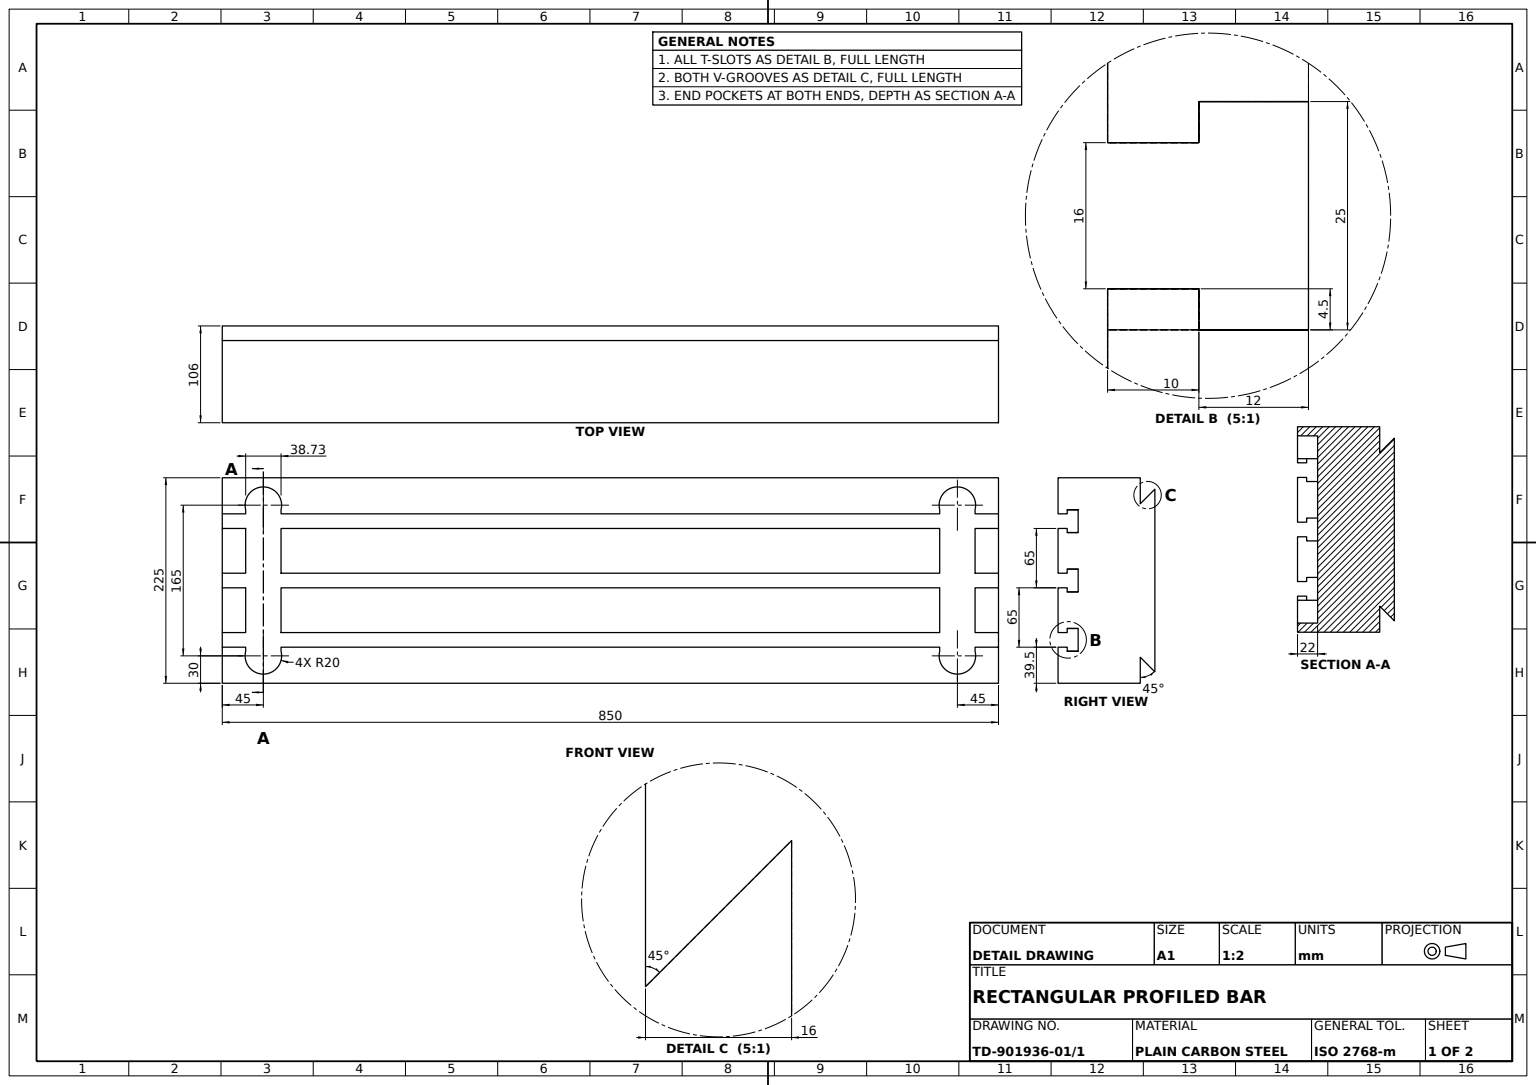
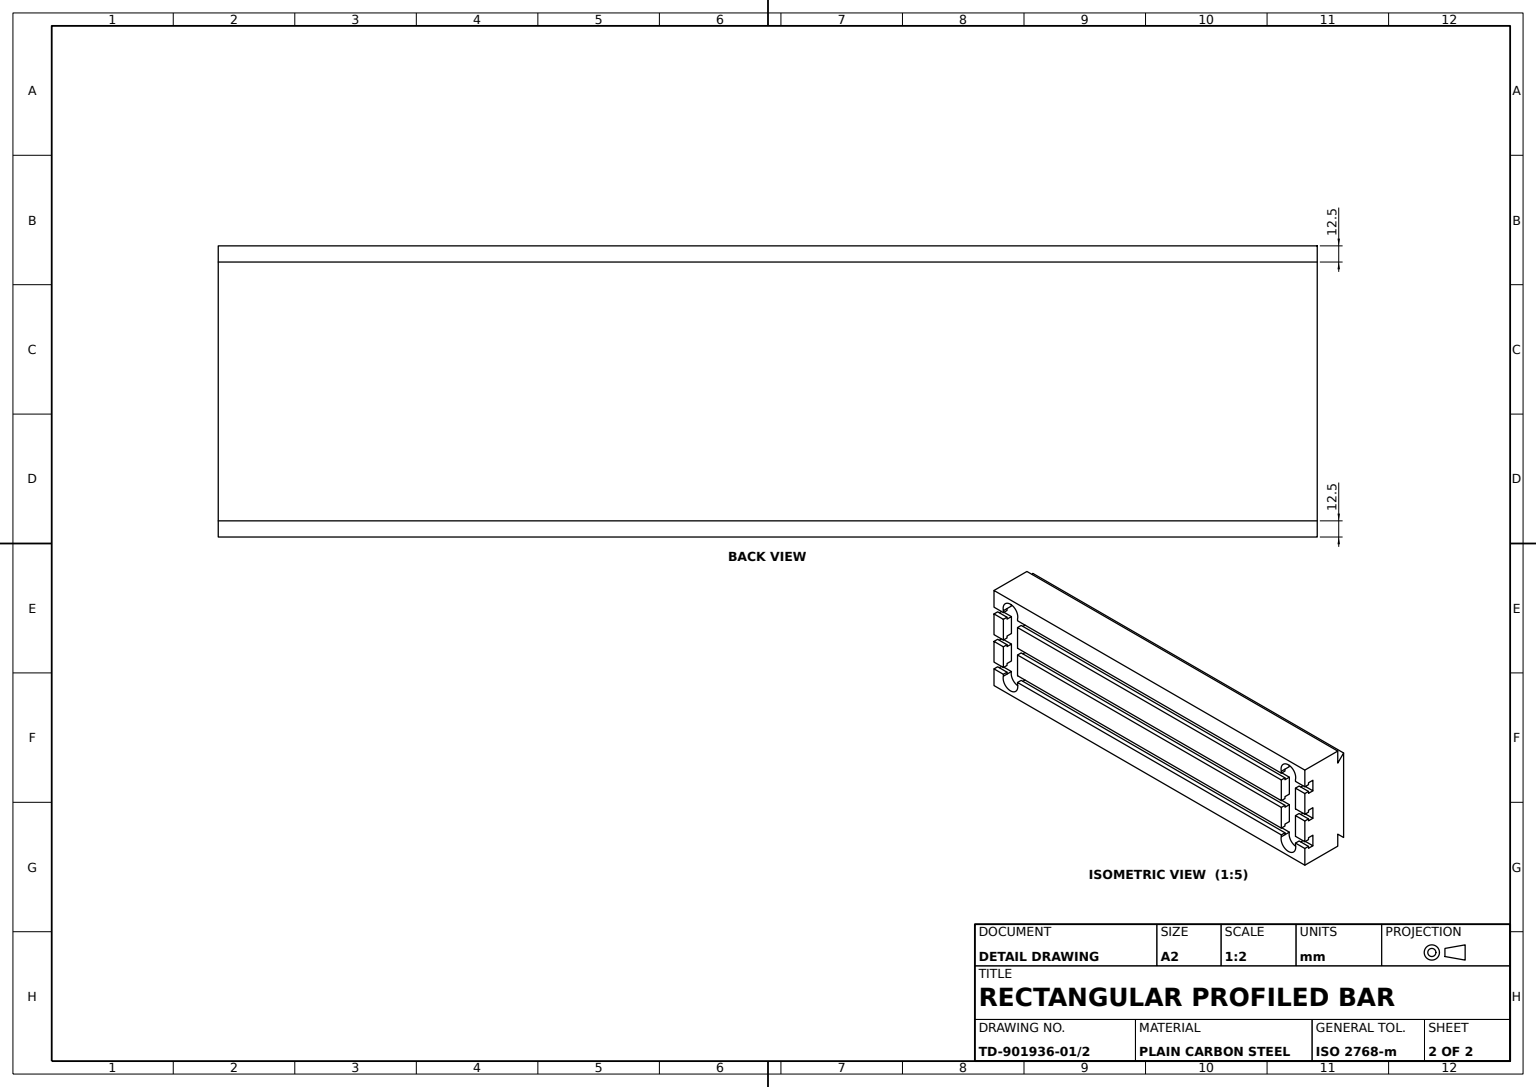
solid
v1 (-400,82.5,106)
v2 (-399.363172,77.493249,106)
e1 v1 v2 CIRCLE(AX(P(-380,82.5,106),D(0,0,1),D(1,0,0)),20)
v3 (-399.363172,77.493249,96)
e2 v3 v2 LINE
v4 (-399.364917,77.5,96)
e3 v4 v3 CIRCLE(AX(P(-380,82.5,96),D(0,0,1),D(1,0,0)),20)
v5 (-399.364917,77.5,84)
e4 v5 v4 LINE
v6 (-400,82.5,84)
e5 v6 v5 CIRCLE(AX(P(-380,82.5,84),D(0,0,1),D(-1,0,0)),20)
e6 v6 v1 LINE
face CYL(AX(P(-380,82.5,-124.865986),D(0,0,1),D(1,0,0)),20) rev [e1 -e2 -e3 -e4 -e5 e6]
v7 (360.635083,-77.5,96)
v8 (360.635083,-77.5,84)
e7 v7 v8 LINE
v9 (-360.635083,-77.5,84)
e8 v9 v8 LINE
v10 (-360.635083,-77.5,96)
e9 v9 v10 LINE
e10 v10 v7 LINE
face PLANE(AX(P(-425,-77.5,96),D(0,-1,0),D(0,0,-1))) rev [e7 -e8 e9 e10]
v11 (-400,-82.5,106)
v12 (-360,-82.5,106)
e11 v11 v12 CIRCLE(AX(P(-380,-82.5,106),D(0,0,1),D(1,0,0)),20)
v13 (-399.363172,-77.493249,106)
e12 v13 v11 CIRCLE(AX(P(-380,-82.5,106),D(0,0,1),D(1,0,0)),20)
v14 (-399.363172,-73,106)
e13 v14 v13 LINE
v15 (-425,-73,106)
e14 v15 v14 LINE
v16 (-425,-112.5,106)
e15 v15 v16 LINE
v17 (425,-112.5,106)
e16 v16 v17 LINE
v18 (425,-73,106)
e17 v17 v18 LINE
v19 (399.363172,-73,106)
e18 v19 v18 LINE
v20 (399.363172,-77.493249,106)
e19 v20 v19 LINE
v21 (400,-82.5,106)
e20 v21 v20 CIRCLE(AX(P(380,-82.5,106),D(0,0,1),D(-1,0,0)),20)
v22 (360,-82.5,106)
e21 v22 v21 CIRCLE(AX(P(380,-82.5,106),D(0,0,1),D(-1,0,0)),20)
v23 (360.636828,-77.493249,106)
e22 v23 v22 CIRCLE(AX(P(380,-82.5,106),D(0,0,1),D(-1,0,0)),20)
v24 (360.636828,-73,106)
e23 v24 v23 LINE
v25 (-360.636828,-73,106)
e24 v25 v24 LINE
v26 (-360.636828,-77.493249,106)
e25 v26 v25 LINE
e26 v12 v26 CIRCLE(AX(P(-380,-82.5,106),D(0,0,1),D(1,0,0)),20)
face PLANE(AX(P(0,0,106),D(0,0,1),D(1,0,0))) [-e11 -e12 -e13 -e14 e15 e16 e17 -e18 -e19 -e20 -e21 -e22 -e23 -e24 -e25 -e26]
v27 (-425,-8,106)
v28 (-425,-57,106)
e27 v27 v28 LINE
v29 (-425,-8,96)
e28 v27 v29 LINE
v30 (-425,-12.5,96)
e29 v29 v30 LINE
v31 (-425,-12.5,84)
e30 v30 v31 LINE
v32 (-425,12.5,84)
e31 v31 v32 LINE
v33 (-425,12.5,96)
e32 v32 v33 LINE
v34 (-425,8,96)
e33 v33 v34 LINE
v35 (-425,8,106)
e34 v34 v35 LINE
v36 (-425,57,106)
e35 v36 v35 LINE
v37 (-425,57,96)
e36 v36 v37 LINE
v38 (-425,52.5,96)
e37 v37 v38 LINE
v39 (-425,52.5,84)
e38 v38 v39 LINE
v40 (-425,77.5,84)
e39 v39 v40 LINE
v41 (-425,77.5,96)
e40 v40 v41 LINE
v42 (-425,73,96)
e41 v41 v42 LINE
v43 (-425,73,106)
e42 v42 v43 LINE
v44 (-425,112.5,106)
e43 v44 v43 LINE
v45 (-425,112.5,16)
e44 v44 v45 LINE
v46 (-425,84,16)
e45 v45 v46 LINE
v47 (-425,100,0)
e46 v46 v47 LINE
v48 (-425,-100,0)
e47 v47 v48 LINE
v49 (-425,-84,16)
e48 v48 v49 LINE
v50 (-425,-112.5,16)
e49 v49 v50 LINE
e50 v16 v50 LINE
v51 (-425,-73,96)
e51 v15 v51 LINE
v52 (-425,-77.5,96)
e52 v51 v52 LINE
v53 (-425,-77.5,84)
e53 v52 v53 LINE
v54 (-425,-52.5,84)
e54 v53 v54 LINE
v55 (-425,-52.5,96)
e55 v54 v55 LINE
v56 (-425,-57,96)
e56 v55 v56 LINE
e57 v56 v28 LINE
face PLANE(AX(P(-425,-112.5,106),D(1,0,0),D(0,0,-1))) rev [-e27 e28 e29 e30 e31 e32 e33 e34 -e35 e36 e37 e38 e39 e40 e41 e42 -e43 e44 e45 e46 e47 e48 e49 -e50 -e15 e51 e52 e53 e54 e55 e56 e57]
v57 (399.363172,-12.5,96)
v58 (399.363172,-8,96)
e58 v57 v58 LINE
v59 (425,-8,96)
e59 v58 v59 LINE
v60 (425,-12.5,96)
e60 v59 v60 LINE
e61 v57 v60 LINE
face PLANE(AX(P(-425,-8,96),D(0,0,1),D(1,0,0))) rev [e58 e59 e60 -e61]
v61 (425,-84,16)
e62 v49 v61 LINE
v62 (425,-112.5,16)
e63 v61 v62 LINE
e64 v50 v62 LINE
face PLANE(AX(P(-425,-84,16),D(0,0,1),D(0,-1,0))) rev [-e49 e62 e63 -e64]
v63 (-360,-82.5,84)
e65 v63 v12 LINE
v64 (-400,-82.5,84)
e66 v64 v63 CIRCLE(AX(P(-380,-82.5,84),D(0,0,1),D(-1,0,0)),20)
e67 v64 v11 LINE
face CYL(AX(P(-380,-82.5,-124.865986),D(0,0,1),D(1,0,0)),20) rev [e11 -e65 -e66 e67]
v65 (-399.364917,-77.5,96)
e68 v52 v65 LINE
v66 (-399.364917,-77.5,84)
e69 v65 v66 LINE
e70 v53 v66 LINE
face PLANE(AX(P(-425,-77.5,96),D(0,-1,0),D(0,0,-1))) rev [e68 e69 -e70 -e53]
e71 v17 v62 LINE
face PLANE(AX(P(425,-112.5,106),D(0,1,0),D(-1,0,0))) rev [e50 e64 -e71 -e16]
v67 (-399.363172,73,96)
e72 v3 v67 LINE
v68 (-399.363172,73,106)
e73 v2 v68 LINE
e74 v67 v68 LINE
face PLANE(AX(P(-399.363172,-77.493249,-124.865986),D(-1,0,0),D(0,0,1))) rev [-e72 e2 e73 -e74]
v69 (399.363172,73,96)
v70 (399.363172,77.493249,96)
e75 v69 v70 LINE
v71 (399.364917,77.5,96)
e76 v70 v71 CIRCLE(AX(P(380,82.5,96),D(0,0,1),D(1,0,0)),20)
v72 (425,77.5,96)
e77 v71 v72 LINE
v73 (425,73,96)
e78 v72 v73 LINE
e79 v69 v73 LINE
face PLANE(AX(P(-425,73,96),D(0,0,1),D(1,0,0))) rev [e75 e76 e77 e78 -e79]
v74 (399.363172,57,96)
v75 (425,57,96)
e80 v74 v75 LINE
v76 (399.363172,57,106)
e81 v74 v76 LINE
v77 (425,57,106)
e82 v76 v77 LINE
e83 v77 v75 LINE
face PLANE(AX(P(-425,57,106),D(0,-1,0),D(0,0,-1))) rev [-e80 e81 e82 e83]
v78 (360.636828,57,106)
v79 (360.636828,8,106)
e84 v78 v79 LINE
v80 (360.636828,8,96)
e85 v80 v79 LINE
v81 (360.636828,12.5,96)
e86 v81 v80 LINE
v82 (360.636828,12.5,84)
e87 v82 v81 LINE
v83 (360.636828,52.5,84)
e88 v83 v82 LINE
v84 (360.636828,52.5,96)
e89 v84 v83 LINE
v85 (360.636828,57,96)
e90 v85 v84 LINE
e91 v78 v85 LINE
face PLANE(AX(P(360.636828,-77.493249,-124.865986),D(-1,0,0),D(0,0,1))) rev [e84 -e85 -e86 -e87 -e88 -e89 -e90 -e91]
v86 (360.636828,-77.493249,96)
e92 v86 v23 LINE
v87 (360.636828,-73,96)
e93 v87 v86 LINE
e94 v24 v87 LINE
face PLANE(AX(P(360.636828,-77.493249,-124.865986),D(-1,0,0),D(0,0,1))) rev [e23 -e92 -e93 -e94]
v88 (399.363172,-52.5,84)
v89 (425,-52.5,84)
e95 v88 v89 LINE
v90 (425,-52.5,96)
e96 v89 v90 LINE
v91 (399.363172,-52.5,96)
e97 v91 v90 LINE
e98 v91 v88 LINE
face PLANE(AX(P(-425,-52.5,96),D(0,1,0),D(0,0,1))) rev [e95 e96 -e97 e98]
v92 (-399.363172,8,96)
e99 v34 v92 LINE
v93 (-399.363172,8,106)
e100 v92 v93 LINE
e101 v35 v93 LINE
face PLANE(AX(P(-425,8,106),D(0,1,0),D(0,0,1))) rev [e99 e100 -e101 -e34]
v94 (425,12.5,96)
v95 (425,8,96)
e102 v94 v95 LINE
v96 (399.363172,8,96)
e103 v96 v95 LINE
v97 (399.363172,12.5,96)
e104 v96 v97 LINE
e105 v97 v94 LINE
face PLANE(AX(P(-425,8,96),D(0,0,1),D(1,0,0))) rev [e102 -e103 e104 e105]
v98 (425,112.5,16)
v99 (425,84,16)
e106 v98 v99 LINE
e107 v46 v99 LINE
e108 v45 v98 LINE
face PLANE(AX(P(-425,84,16),D(0,0,1),D(0,-1,0))) rev [e106 -e107 -e45 e108]
v100 (425,52.5,96)
e109 v75 v100 LINE
v101 (399.363172,52.5,96)
e110 v101 v100 LINE
e111 v101 v74 LINE
face PLANE(AX(P(-425,57,96),D(0,0,1),D(1,0,0))) rev [e109 -e110 e111 e80]
v102 (360.636828,-8,96)
v103 (360.636828,-12.5,96)
e112 v102 v103 LINE
v104 (-360.636828,-12.5,96)
e113 v104 v103 LINE
v105 (-360.636828,-8,96)
e114 v104 v105 LINE
e115 v105 v102 LINE
face PLANE(AX(P(-425,-8,96),D(0,0,1),D(1,0,0))) rev [e112 -e113 e114 e115]
v106 (-399.363172,-77.493249,96)
e116 v106 v13 LINE
e117 v66 v64 CIRCLE(AX(P(-380,-82.5,84),D(0,0,1),D(-1,0,0)),20)
e118 v106 v65 CIRCLE(AX(P(-380,-82.5,96),D(0,0,1),D(1,0,0)),20)
face CYL(AX(P(-380,-82.5,-124.865986),D(0,0,1),D(1,0,0)),20) rev [e116 e12 -e67 -e117 -e69 -e118]
v107 (400,82.5,84)
v108 (400,82.5,106)
e119 v107 v108 LINE
v109 (360,82.5,106)
e120 v108 v109 CIRCLE(AX(P(380,82.5,106),D(0,0,1),D(-1,0,0)),20)
v110 (360,82.5,84)
e121 v110 v109 LINE
e122 v107 v110 CIRCLE(AX(P(380,82.5,84),D(0,0,1),D(-1,0,0)),20)
face CYL(AX(P(380,82.5,-124.865986),D(0,0,1),D(1,0,0)),20) rev [e119 e120 -e121 -e122]
v111 (425,100,0)
e123 v99 v111 LINE
e124 v47 v111 LINE
face PLANE(AX(P(-425,100,0),D(0,-0.707106781,-0.707106781),D(0,0.707106781,-0.707106781))) rev [-e46 e107 e123 -e124]
v112 (-399.363172,57,106)
e125 v112 v93 LINE
e126 v36 v112 LINE
face PLANE(AX(P(0,0,106),D(0,0,1),D(1,0,0))) [e101 -e125 -e126 e35]
v113 (-399.363172,-8,96)
e127 v29 v113 LINE
v114 (-399.363172,-12.5,96)
e128 v113 v114 LINE
e129 v30 v114 LINE
face PLANE(AX(P(-425,-8,96),D(0,0,1),D(1,0,0))) rev [e127 e128 -e129 -e29]
v115 (-360.636828,57,106)
e130 v115 v78 LINE
v116 (-360.636828,8,106)
e131 v116 v115 LINE
e132 v116 v79 LINE
face PLANE(AX(P(0,0,106),D(0,0,1),D(1,0,0))) [-e130 -e131 e132 -e84]
v117 (360,-82.5,84)
e133 v117 v22 LINE
e134 v8 v117 CIRCLE(AX(P(380,-82.5,84),D(0,0,1),D(-1,0,0)),20)
e135 v86 v7 CIRCLE(AX(P(380,-82.5,96),D(0,0,1),D(1,0,0)),20)
face CYL(AX(P(380,-82.5,-124.865986),D(0,0,1),D(1,0,0)),20) rev [e22 -e133 -e134 -e7 -e135 e92]
v118 (-360.636828,-12.5,84)
v119 (360.636828,-12.5,84)
e136 v118 v119 LINE
e137 v118 v104 LINE
e138 v103 v119 LINE
face PLANE(AX(P(-425,-12.5,96),D(0,-1,0),D(0,0,-1))) rev [-e136 e137 e113 e138]
v120 (-360.636828,8,96)
e139 v120 v80 LINE
v121 (-360.636828,12.5,96)
e140 v120 v121 LINE
e141 v121 v81 LINE
face PLANE(AX(P(-425,8,96),D(0,0,1),D(1,0,0))) rev [e86 -e139 e140 e141]
v122 (425,-100,0)
e142 v122 v61 LINE
e143 v48 v122 LINE
face PLANE(AX(P(-425,-100,0),D(0,0.707106781,-0.707106781),D(0,0.707106781,0.707106781))) rev [e142 -e62 -e48 e143]
v123 (399.363172,-73,96)
e144 v123 v19 LINE
v124 (399.363172,-77.493249,96)
e145 v124 v123 LINE
e146 v124 v20 LINE
face PLANE(AX(P(399.363172,-77.493249,-124.865986),D(1,0,0),D(0,0,-1))) rev [-e144 -e145 e146 e19]
v125 (-399.363172,57,96)
e147 v112 v125 LINE
v126 (-399.363172,12.5,96)
e148 v126 v92 LINE
v127 (-399.363172,12.5,84)
e149 v127 v126 LINE
v128 (-399.363172,52.5,84)
e150 v128 v127 LINE
v129 (-399.363172,52.5,96)
e151 v129 v128 LINE
e152 v125 v129 LINE
face PLANE(AX(P(-399.363172,-77.493249,-124.865986),D(-1,0,0),D(0,0,1))) rev [-e147 e125 -e100 -e148 -e149 -e150 -e151 -e152]
v130 (-360.636828,-52.5,96)
v131 (360.636828,-52.5,96)
e153 v130 v131 LINE
v132 (-360.636828,-52.5,84)
e154 v130 v132 LINE
v133 (360.636828,-52.5,84)
e155 v132 v133 LINE
e156 v133 v131 LINE
face PLANE(AX(P(-425,-52.5,96),D(0,1,0),D(0,0,1))) rev [-e153 e154 e155 e156]
v134 (399.363172,-57,106)
v135 (425,-57,106)
e157 v134 v135 LINE
v136 (399.363172,-57,96)
e158 v134 v136 LINE
v137 (425,-57,96)
e159 v136 v137 LINE
e160 v137 v135 LINE
face PLANE(AX(P(-425,-57,106),D(0,1,0),D(0,0,1))) rev [-e157 e158 e159 e160]
v138 (-399.363172,-12.5,84)
e161 v114 v138 LINE
e162 v31 v138 LINE
face PLANE(AX(P(-425,-12.5,96),D(0,-1,0),D(0,0,-1))) rev [e129 e161 -e162 -e30]
v139 (399.364917,-77.5,96)
v140 (425,-77.5,96)
e163 v139 v140 LINE
e164 v139 v124 CIRCLE(AX(P(380,-82.5,96),D(0,0,1),D(1,0,0)),20)
v141 (425,-73,96)
e165 v123 v141 LINE
e166 v141 v140 LINE
face PLANE(AX(P(-425,-73,96),D(0,0,1),D(1,0,0))) rev [-e163 e164 e145 e165 e166]
v142 (425,73,106)
v143 (425,112.5,106)
e167 v142 v143 LINE
e168 v143 v44 LINE
e169 v43 v68 LINE
v144 (-360,82.5,106)
e170 v144 v1 CIRCLE(AX(P(-380,82.5,106),D(0,0,1),D(1,0,0)),20)
v145 (-360.636828,77.493249,106)
e171 v145 v144 CIRCLE(AX(P(-380,82.5,106),D(0,0,1),D(1,0,0)),20)
v146 (-360.636828,73,106)
e172 v146 v145 LINE
v147 (360.636828,73,106)
e173 v146 v147 LINE
v148 (360.636828,77.493249,106)
e174 v148 v147 LINE
e175 v109 v148 CIRCLE(AX(P(380,82.5,106),D(0,0,1),D(-1,0,0)),20)
v149 (399.363172,77.493249,106)
e176 v149 v108 CIRCLE(AX(P(380,82.5,106),D(0,0,1),D(-1,0,0)),20)
v150 (399.363172,73,106)
e177 v150 v149 LINE
e178 v150 v142 LINE
face PLANE(AX(P(0,0,106),D(0,0,1),D(1,0,0))) [e167 e168 e43 e169 -e73 -e1 -e170 -e171 -e172 e173 -e174 -e175 -e120 -e176 -e177 e178]
v151 (-360.636828,57,96)
e179 v151 v85 LINE
e180 v151 v115 LINE
face PLANE(AX(P(-425,57,106),D(0,-1,0),D(0,0,-1))) rev [-e179 e180 e130 e91]
v152 (-360.636828,52.5,96)
e181 v152 v151 LINE
v153 (-360.636828,52.5,84)
e182 v153 v152 LINE
v154 (-360.636828,12.5,84)
e183 v154 v153 LINE
e184 v121 v154 LINE
e185 v116 v120 LINE
face PLANE(AX(P(-360.636828,-77.493249,-124.865986),D(1,0,0),D(0,0,-1))) rev [-e180 -e181 -e182 -e183 -e184 -e140 -e185 e131]
e186 v152 v84 LINE
face PLANE(AX(P(-425,57,96),D(0,0,1),D(1,0,0))) rev [-e186 e181 e179 e90]
e187 v37 v125 LINE
face PLANE(AX(P(-425,57,106),D(0,-1,0),D(0,0,-1))) rev [e126 e147 -e187 -e36]
v155 (-399.363172,-57,96)
e188 v56 v155 LINE
v156 (-399.363172,-57,106)
e189 v155 v156 LINE
e190 v28 v156 LINE
face PLANE(AX(P(-425,-57,106),D(0,1,0),D(0,0,1))) rev [-e57 e188 e189 -e190]
v157 (360.635083,77.5,84)
e191 v110 v157 CIRCLE(AX(P(380,82.5,84),D(0,0,1),D(-1,0,0)),20)
v158 (360.636828,77.493249,96)
e192 v158 v148 LINE
v159 (360.635083,77.5,96)
e193 v159 v158 CIRCLE(AX(P(380,82.5,96),D(0,0,1),D(1,0,0)),20)
e194 v157 v159 LINE
face CYL(AX(P(380,82.5,-124.865986),D(0,0,1),D(1,0,0)),20) rev [-e191 e121 e175 -e192 -e193 -e194]
v160 (425,12.5,84)
e195 v160 v94 LINE
v161 (399.363172,12.5,84)
e196 v97 v161 LINE
e197 v161 v160 LINE
face PLANE(AX(P(-425,12.5,96),D(0,1,0),D(0,0,1))) rev [e195 -e105 e196 e197]
e198 v150 v69 LINE
e199 v70 v149 LINE
face PLANE(AX(P(399.363172,-77.493249,-124.865986),D(1,0,0),D(0,0,-1))) rev [-e198 e177 -e199 -e75]
e200 v42 v67 LINE
e201 v41 v4 LINE
face PLANE(AX(P(-425,73,96),D(0,0,1),D(1,0,0))) rev [e72 -e200 -e41 e201 e3]
v162 (-360.636828,-77.493249,96)
e202 v10 v162 CIRCLE(AX(P(-380,-82.5,96),D(0,0,1),D(1,0,0)),20)
v163 (-360.636828,-73,96)
e203 v162 v163 LINE
e204 v163 v87 LINE
face PLANE(AX(P(-425,-73,96),D(0,0,1),D(1,0,0))) rev [-e10 e202 e203 e204 e93 e135]
v164 (360.636828,-57,96)
v165 (360.636828,-57,106)
e205 v164 v165 LINE
e206 v131 v164 LINE
e207 v119 v133 LINE
v166 (360.636828,-8,106)
e208 v166 v102 LINE
e209 v166 v165 LINE
face PLANE(AX(P(360.636828,-77.493249,-124.865986),D(-1,0,0),D(0,0,1))) rev [-e205 -e206 -e156 -e207 -e138 -e112 -e208 e209]
e210 v40 v5 LINE
face PLANE(AX(P(-425,77.5,96),D(0,1,0),D(0,0,1))) rev [e4 -e201 -e40 e210]
v167 (399.363172,8,106)
e211 v167 v76 LINE
v168 (425,8,106)
e212 v167 v168 LINE
e213 v168 v77 LINE
face PLANE(AX(P(0,0,106),D(0,0,1),D(1,0,0))) [-e211 e212 e213 -e82]
v169 (-399.363172,-8,106)
e214 v169 v156 LINE
v170 (-399.363172,-52.5,96)
e215 v170 v155 LINE
v171 (-399.363172,-52.5,84)
e216 v171 v170 LINE
e217 v138 v171 LINE
e218 v169 v113 LINE
face PLANE(AX(P(-399.363172,-77.493249,-124.865986),D(-1,0,0),D(0,0,1))) rev [e214 -e189 -e215 -e216 -e217 -e161 -e128 -e218]
e219 v163 v25 LINE
face PLANE(AX(P(-425,-73,106),D(0,-1,0),D(0,0,-1))) rev [e24 e94 -e204 e219]
v172 (399.364917,-77.5,84)
e220 v172 v139 LINE
v173 (425,-77.5,84)
e221 v140 v173 LINE
e222 v172 v173 LINE
face PLANE(AX(P(-425,-77.5,96),D(0,-1,0),D(0,0,-1))) rev [e220 e163 e221 -e222]
v174 (-360.635083,77.5,84)
v175 (-360,82.5,84)
e223 v174 v175 CIRCLE(AX(P(-380,82.5,84),D(0,0,1),D(-1,0,0)),20)
v176 (-360.635083,77.5,96)
e224 v176 v174 LINE
v177 (-360.636828,77.493249,96)
e225 v177 v176 CIRCLE(AX(P(-380,82.5,96),D(0,0,1),D(1,0,0)),20)
e226 v177 v145 LINE
e227 v175 v144 LINE
face CYL(AX(P(-380,82.5,-124.865986),D(0,0,1),D(1,0,0)),20) rev [-e223 -e224 -e225 e226 e171 -e227]
face PLANE(AX(P(-425,8,106),D(0,1,0),D(0,0,1))) rev [e185 e139 e85 -e132]
v178 (-360.636828,-8,106)
e228 v178 v166 LINE
v179 (-360.636828,-57,106)
e229 v179 v178 LINE
e230 v179 v165 LINE
face PLANE(AX(P(0,0,106),D(0,0,1),D(1,0,0))) [-e228 -e229 e230 -e209]
e231 v73 v142 LINE
face PLANE(AX(P(-425,73,106),D(0,1,0),D(0,0,1))) rev [e198 e79 e231 -e178]
e232 v136 v91 LINE
e233 v90 v137 LINE
face PLANE(AX(P(-425,-57,96),D(0,0,1),D(1,0,0))) rev [-e159 e232 e97 e233]
e234 v167 v96 LINE
v180 (399.363172,52.5,84)
e235 v180 v101 LINE
e236 v161 v180 LINE
face PLANE(AX(P(399.363172,-77.493249,-124.865986),D(1,0,0),D(0,0,-1))) rev [-e234 e211 -e81 -e111 -e235 -e236 -e196 -e104]
e237 v176 v159 LINE
e238 v174 v157 LINE
face PLANE(AX(P(-425,77.5,96),D(0,1,0),D(0,0,1))) rev [-e237 e224 e238 e194]
v181 (399.363172,-8,106)
e239 v58 v181 LINE
v182 (399.363172,-12.5,84)
e240 v182 v57 LINE
e241 v88 v182 LINE
e242 v134 v181 LINE
face PLANE(AX(P(399.363172,-77.493249,-124.865986),D(1,0,0),D(0,0,-1))) rev [-e239 -e58 -e240 -e241 -e98 -e232 -e158 e242]
e243 v39 v128 LINE
e244 v32 v127 LINE
e245 v54 v171 LINE
e246 v63 v9 CIRCLE(AX(P(-380,-82.5,84),D(0,0,1),D(-1,0,0)),20)
v183 (400,-82.5,84)
e247 v117 v183 CIRCLE(AX(P(380,-82.5,84),D(0,0,1),D(-1,0,0)),20)
e248 v183 v172 CIRCLE(AX(P(380,-82.5,84),D(0,0,1),D(-1,0,0)),20)
e249 v173 v89 LINE
v184 (425,-12.5,84)
e250 v182 v184 LINE
e251 v184 v160 LINE
v185 (425,52.5,84)
e252 v180 v185 LINE
v186 (425,77.5,84)
e253 v185 v186 LINE
v187 (399.364917,77.5,84)
e254 v187 v186 LINE
e255 v187 v107 CIRCLE(AX(P(380,82.5,84),D(0,0,1),D(-1,0,0)),20)
e256 v175 v6 CIRCLE(AX(P(-380,82.5,84),D(0,0,1),D(-1,0,0)),20)
e257 v154 v82 LINE
e258 v153 v83 LINE
e259 v132 v118 LINE
face PLANE(AX(P(-425,77.5,84),D(0,0,-1),D(0,1,0))) rev [-e210 -e39 e243 e150 -e244 -e31 e162 e217 -e245 -e54 e70 e117 e66 e246 e8 e134 e247 e248 e222 e249 -e95 e241 e250 e251 -e197 e236 e252 e253 -e254 e255 e122 e191 -e238 e223 e256 e5] [-e257 e183 e258 e88] [e259 e136 e207 -e155]
e260 v33 v126 LINE
face PLANE(AX(P(-425,12.5,96),D(0,1,0),D(0,0,1))) rev [-e260 -e32 e244 e149]
v188 (-360.636828,-57,96)
e261 v188 v164 LINE
e262 v179 v188 LINE
face PLANE(AX(P(-425,-57,106),D(0,1,0),D(0,0,1))) rev [e261 e205 -e230 e262]
e263 v183 v21 LINE
face CYL(AX(P(380,-82.5,-124.865986),D(0,0,1),D(1,0,0)),20) rev [e21 -e263 -e247 e133]
e264 v27 v169 LINE
face PLANE(AX(P(-425,-8,106),D(0,-1,0),D(0,0,-1))) rev [-e28 e264 e218 -e127]
e265 v122 v111 LINE
face PLANE(AX(P(0,0,0),D(0,0,1),D(1,0,0))) rev [-e47 e124 -e265 -e143]
v189 (-360.636828,73,96)
e266 v146 v189 LINE
e267 v189 v177 LINE
face PLANE(AX(P(-360.636828,-77.493249,-124.865986),D(1,0,0),D(0,0,-1))) rev [-e266 e172 -e226 -e267]
e268 v71 v187 LINE
face CYL(AX(P(380,82.5,-124.865986),D(0,0,1),D(1,0,0)),20) rev [-e255 -e268 -e76 e199 e176 -e119]
v190 (425,-8,106)
e269 v181 v190 LINE
e270 v135 v190 LINE
face PLANE(AX(P(0,0,106),D(0,0,1),D(1,0,0))) [-e269 -e242 e157 e270]
e271 v55 v170 LINE
face PLANE(AX(P(-425,-52.5,96),D(0,1,0),D(0,0,1))) rev [e216 -e271 -e55 e245]
face PLANE(AX(P(-425,8,96),D(0,0,1),D(1,0,0))) rev [e260 e148 -e99 -e33]
e272 v162 v26 LINE
face CYL(AX(P(-380,-82.5,-124.865986),D(0,0,1),D(1,0,0)),20) rev [-e246 e65 e26 -e272 -e202 -e9]
e273 v38 v129 LINE
face PLANE(AX(P(-425,57,96),D(0,0,1),D(1,0,0))) rev [-e273 -e37 e187 e152]
e274 v105 v178 LINE
face PLANE(AX(P(-425,-8,106),D(0,-1,0),D(0,0,-1))) rev [e274 e228 e208 -e115]
v191 (360.636828,73,96)
e275 v189 v191 LINE
e276 v191 v147 LINE
face PLANE(AX(P(-425,73,106),D(0,1,0),D(0,0,1))) rev [-e173 e266 e275 e276]
v192 (-399.363172,-73,96)
e277 v51 v192 LINE
e278 v192 v106 LINE
face PLANE(AX(P(-425,-73,96),D(0,0,1),D(1,0,0))) rev [-e52 e277 e278 e118 -e68]
face CYL(AX(P(380,-82.5,-124.865986),D(0,0,1),D(1,0,0)),20) rev [e20 -e146 -e164 -e220 -e248 e263]
e279 v14 v192 LINE
face PLANE(AX(P(-399.363172,-77.493249,-124.865986),D(-1,0,0),D(0,0,1))) rev [e13 -e116 -e278 -e279]
e280 v186 v72 LINE
face PLANE(AX(P(-425,77.5,96),D(0,1,0),D(0,0,1))) rev [e280 -e77 e268 e254]
face CYL(AX(P(-380,82.5,-124.865986),D(0,0,1),D(1,0,0)),20) rev [e227 e170 -e6 -e256]
face PLANE(AX(P(-425,-57,96),D(0,0,1),D(1,0,0))) rev [e271 e215 -e188 -e56]
e281 v158 v191 LINE
face PLANE(AX(P(-425,73,96),D(0,0,1),D(1,0,0))) rev [-e275 e267 e225 e237 e193 e281]
e282 v188 v130 LINE
face PLANE(AX(P(-360.636828,-77.493249,-124.865986),D(1,0,0),D(0,0,-1))) rev [-e274 -e114 -e137 -e259 -e154 -e282 -e262 e229]
e283 v95 v168 LINE
face PLANE(AX(P(-425,8,106),D(0,1,0),D(0,0,1))) rev [e103 e283 -e212 e234]
face PLANE(AX(P(-425,73,106),D(0,1,0),D(0,0,1))) rev [-e42 e200 e74 -e169]
face PLANE(AX(P(-360.636828,-77.493249,-124.865986),D(1,0,0),D(0,0,-1))) rev [e272 e25 -e219 -e203]
face PLANE(AX(P(-425,52.5,96),D(0,-1,0),D(0,0,-1))) rev [e273 e151 -e243 -e38]
face PLANE(AX(P(360.636828,-77.493249,-124.865986),D(-1,0,0),D(0,0,1))) rev [-e276 -e281 e192 e174]
e284 v190 v59 LINE
face PLANE(AX(P(-425,-8,106),D(0,-1,0),D(0,0,-1))) rev [e239 e269 e284 -e59]
e285 v18 v141 LINE
face PLANE(AX(P(-425,-73,106),D(0,-1,0),D(0,0,-1))) rev [e285 -e165 e144 e18]
face PLANE(AX(P(-425,-57,96),D(0,0,1),D(1,0,0))) rev [e282 e153 e206 -e261]
e286 v100 v185 LINE
face PLANE(AX(P(-425,52.5,96),D(0,-1,0),D(0,0,-1))) rev [-e252 e235 e110 e286]
face PLANE(AX(P(-425,12.5,96),D(0,1,0),D(0,0,1))) rev [e87 -e141 e184 e257]
e287 v143 v98 LINE
face PLANE(AX(P(425,112.5,106),D(0,-1,0),D(1,0,0))) rev [-e108 -e44 -e168 e287]
e288 v60 v184 LINE
face PLANE(AX(P(425,-112.5,106),D(-1,0,0),D(0,0,1))) rev [-e63 -e142 e265 -e123 -e106 -e287 -e167 -e231 -e78 -e280 -e253 -e286 -e109 -e83 -e213 -e283 -e102 -e195 -e251 -e288 -e60 -e284 -e270 -e160 -e233 -e96 -e249 -e221 -e166 -e285 -e17 e71]
face PLANE(AX(P(-425,52.5,96),D(0,-1,0),D(0,0,-1))) rev [e182 e186 e89 -e258]
face PLANE(AX(P(-425,-73,106),D(0,-1,0),D(0,0,-1))) rev [-e51 e14 e279 -e277]
face PLANE(AX(P(-425,-12.5,96),D(0,-1,0),D(0,0,-1))) rev [-e250 e240 e61 e288]
face PLANE(AX(P(0,0,106),D(0,0,1),D(1,0,0))) [-e264 e27 e190 -e214]
